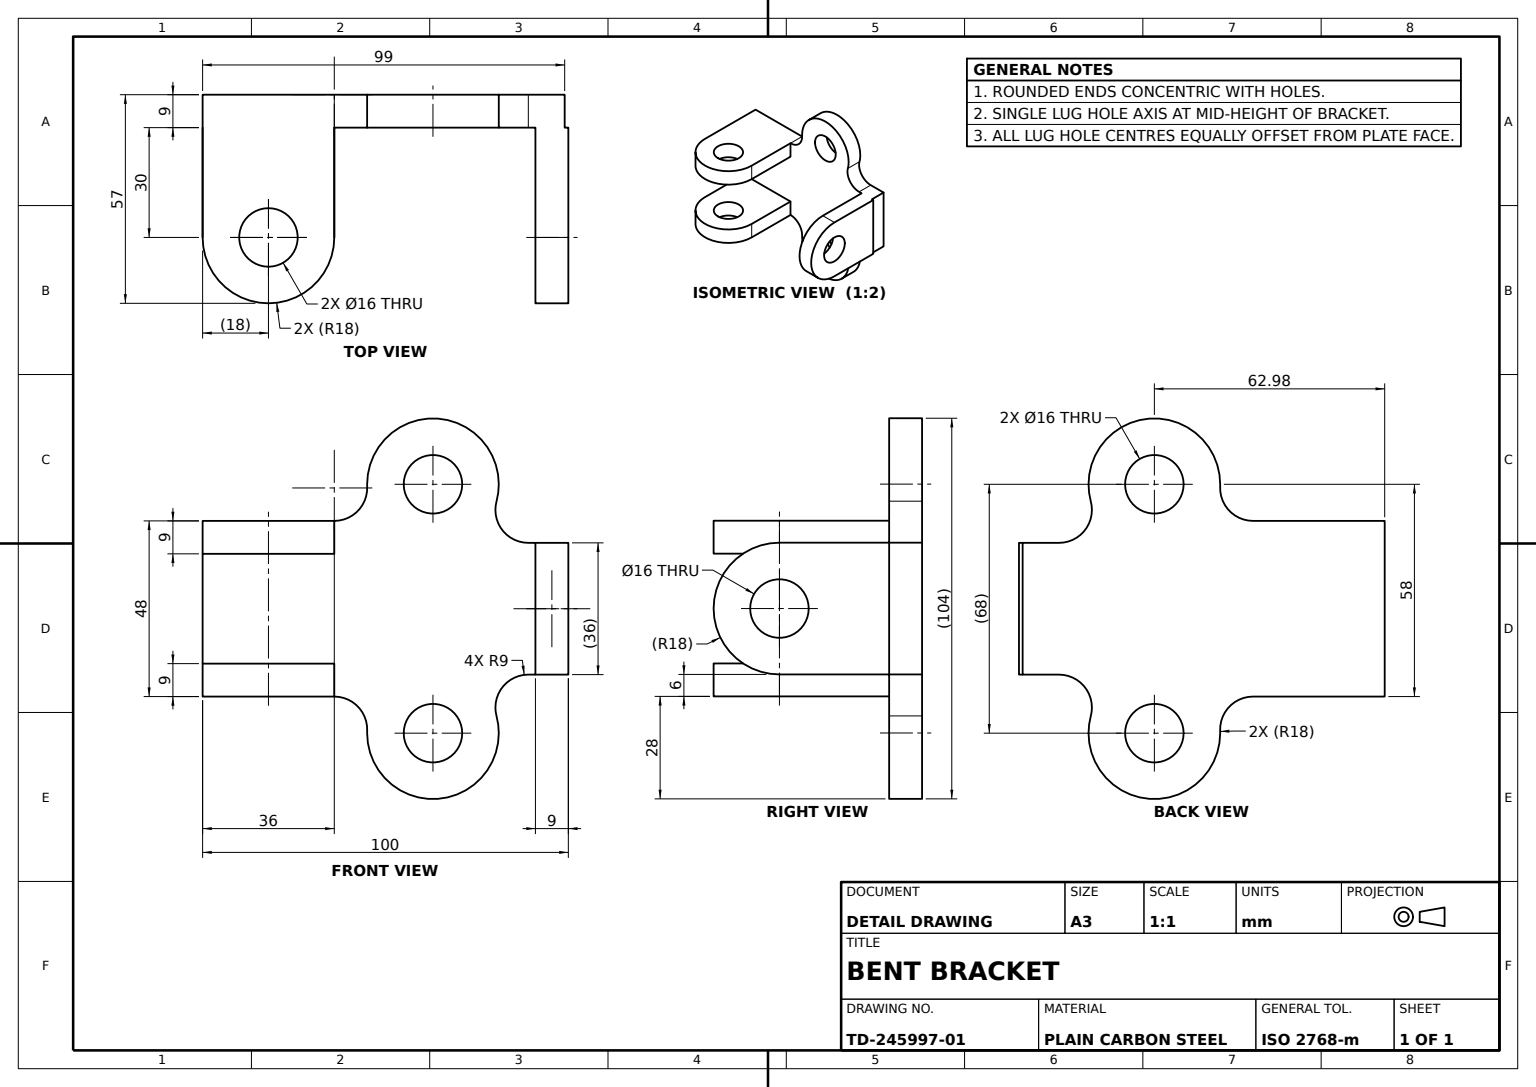
ISO-10303-21;
HEADER;
FILE_DESCRIPTION((''),'2;1');
FILE_NAME('','',(''),(''),'','','');
FILE_SCHEMA(('AUTOMOTIVE_DESIGN'));
ENDSEC;
DATA;
#1=APPLICATION_CONTEXT('');
#2=PRODUCT_CONTEXT('',#1,'mechanical');
#3=PRODUCT('','','',(#2));
#4=PRODUCT_DEFINITION_FORMATION('','',#3);
#5=PRODUCT_DEFINITION_CONTEXT('',#1,'design');
#6=PRODUCT_DEFINITION('','',#4,#5);
#7=PRODUCT_DEFINITION_SHAPE('','',#6);
#8=(LENGTH_UNIT()NAMED_UNIT(*)SI_UNIT(.MILLI.,.METRE.));
#9=(NAMED_UNIT(*)PLANE_ANGLE_UNIT()SI_UNIT($,.RADIAN.));
#10=(NAMED_UNIT(*)SI_UNIT($,.STERADIAN.)SOLID_ANGLE_UNIT());
#11=UNCERTAINTY_MEASURE_WITH_UNIT(LENGTH_MEASURE(1.E-05),#8,'distance_accuracy_value','');
#12=(GEOMETRIC_REPRESENTATION_CONTEXT(3)GLOBAL_UNCERTAINTY_ASSIGNED_CONTEXT((#11))GLOBAL_UNIT_ASSIGNED_CONTEXT((#8,#9,#10))REPRESENTATION_CONTEXT('',''));
#13=CARTESIAN_POINT('',(36.,9.,-30.));
#14=VERTEX_POINT('',#13);
#15=CARTESIAN_POINT('',(36.,0.,-30.));
#16=VERTEX_POINT('',#15);
#17=DIRECTION('',(0.,-1.,0.));
#18=VECTOR('',#17,1000.);
#19=LINE('',#13,#18);
#20=EDGE_CURVE('',#14,#16,#19,.T.);
#21=ORIENTED_EDGE('',*,*,#20,.F.);
#22=CARTESIAN_POINT('',(36.,9.,0.));
#23=VERTEX_POINT('',#22);
#24=DIRECTION('',(0.,0.,-1.));
#25=VECTOR('',#24,1000.);
#26=LINE('',#22,#25);
#27=EDGE_CURVE('',#23,#14,#26,.T.);
#28=ORIENTED_EDGE('',*,*,#27,.F.);
#29=CARTESIAN_POINT('',(36.,0.,0.));
#30=VERTEX_POINT('',#29);
#31=LINE('',#22,#18);
#32=EDGE_CURVE('',#23,#30,#31,.T.);
#33=ORIENTED_EDGE('',*,*,#32,.T.);
#34=LINE('',#29,#25);
#35=EDGE_CURVE('',#30,#16,#34,.T.);
#36=ORIENTED_EDGE('',*,*,#35,.T.);
#37=EDGE_LOOP('',(#21,#28,#33,#36));
#38=FACE_OUTER_BOUND('',#37,.T.);
#39=DIRECTION('',(-1.,0.,0.));
#40=DIRECTION('',(0.,0.,1.));
#41=AXIS2_PLACEMENT_3D('',#22,#39,#40);
#42=PLANE('',#41);
#43=ADVANCED_FACE('',(#38),#42,.F.);
#44=CARTESIAN_POINT('',(91.,24.,-22.));
#45=VERTEX_POINT('',#44);
#46=CARTESIAN_POINT('',(91.,24.,-38.));
#47=VERTEX_POINT('',#46);
#48=CARTESIAN_POINT('',(91.,24.,-30.));
#49=DIRECTION('',(1.,0.,0.));
#50=AXIS2_PLACEMENT_3D('',#48,#49,#24);
#51=CIRCLE('',#50,8.);
#52=EDGE_CURVE('',#45,#47,#51,.T.);
#53=ORIENTED_EDGE('',*,*,#52,.F.);
#54=CARTESIAN_POINT('',(100.,24.,-22.));
#55=VERTEX_POINT('',#54);
#56=VECTOR('',#49,1000.);
#57=LINE('',#44,#56);
#58=EDGE_CURVE('',#45,#55,#57,.T.);
#59=ORIENTED_EDGE('',*,*,#58,.T.);
#60=CARTESIAN_POINT('',(100.,24.,-38.));
#61=VERTEX_POINT('',#60);
#62=CARTESIAN_POINT('',(100.,24.,-30.));
#63=AXIS2_PLACEMENT_3D('',#62,#49,#24);
#64=CIRCLE('',#63,8.);
#65=EDGE_CURVE('',#55,#61,#64,.T.);
#66=ORIENTED_EDGE('',*,*,#65,.T.);
#67=LINE('',#46,#56);
#68=EDGE_CURVE('',#47,#61,#67,.T.);
#69=ORIENTED_EDGE('',*,*,#68,.F.);
#70=EDGE_LOOP('',(#53,#59,#66,#69));
#71=FACE_OUTER_BOUND('',#70,.T.);
#72=CYLINDRICAL_SURFACE('',#50,8.);
#73=ADVANCED_FACE('',(#71),#72,.F.);
#74=CARTESIAN_POINT('',(70.981475,-10.,9.));
#75=VERTEX_POINT('',#74);
#76=CARTESIAN_POINT('',(54.981475,-10.,9.));
#77=VERTEX_POINT('',#76);
#78=CARTESIAN_POINT('',(62.981475,-10.,9.));
#79=AXIS2_PLACEMENT_3D('',#78,#40,#49);
#80=CIRCLE('',#79,8.);
#81=EDGE_CURVE('',#75,#77,#80,.T.);
#82=ORIENTED_EDGE('',*,*,#81,.F.);
#83=EDGE_CURVE('',#77,#75,#80,.T.);
#84=ORIENTED_EDGE('',*,*,#83,.F.);
#85=EDGE_LOOP('',(#82,#84));
#86=FACE_BOUND('',#85,.T.);
#87=CARTESIAN_POINT('',(80.058285,51.,9.));
#88=VERTEX_POINT('',#87);
#89=CARTESIAN_POINT('',(80.366015,53.333333,9.));
#90=VERTEX_POINT('',#89);
#91=CARTESIAN_POINT('',(89.058285,51.,9.));
#92=AXIS2_PLACEMENT_3D('',#91,#24,#49);
#93=CIRCLE('',#92,9.);
#94=EDGE_CURVE('',#88,#90,#93,.T.);
#95=ORIENTED_EDGE('',*,*,#94,.T.);
#96=CARTESIAN_POINT('',(80.981475,58.,9.));
#97=VERTEX_POINT('',#96);
#98=CARTESIAN_POINT('',(62.981475,58.,9.));
#99=AXIS2_PLACEMENT_3D('',#98,#40,#49);
#100=CIRCLE('',#99,18.);
#101=EDGE_CURVE('',#90,#97,#100,.T.);
#102=ORIENTED_EDGE('',*,*,#101,.T.);
#103=CARTESIAN_POINT('',(44.981475,58.,9.));
#104=VERTEX_POINT('',#103);
#105=EDGE_CURVE('',#97,#104,#100,.T.);
#106=ORIENTED_EDGE('',*,*,#105,.T.);
#107=CARTESIAN_POINT('',(44.993825,57.333333,9.));
#108=VERTEX_POINT('',#107);
#109=EDGE_CURVE('',#104,#108,#100,.T.);
#110=ORIENTED_EDGE('',*,*,#109,.T.);
#111=CARTESIAN_POINT('',(36.,48.,9.));
#112=VERTEX_POINT('',#111);
#113=CARTESIAN_POINT('',(36.,57.,9.));
#114=AXIS2_PLACEMENT_3D('',#113,#24,#49);
#115=CIRCLE('',#114,9.);
#116=EDGE_CURVE('',#108,#112,#115,.T.);
#117=ORIENTED_EDGE('',*,*,#116,.T.);
#118=CARTESIAN_POINT('',(0.,48.,9.));
#119=VERTEX_POINT('',#118);
#120=VECTOR('',#39,1000.);
#121=LINE('',#118,#120);
#122=EDGE_CURVE('',#112,#119,#121,.T.);
#123=ORIENTED_EDGE('',*,*,#122,.T.);
#124=CARTESIAN_POINT('',(0.,0.,9.));
#125=VERTEX_POINT('',#124);
#126=LINE('',#124,#18);
#127=EDGE_CURVE('',#119,#125,#126,.T.);
#128=ORIENTED_EDGE('',*,*,#127,.T.);
#129=CARTESIAN_POINT('',(36.,0.,9.));
#130=VERTEX_POINT('',#129);
#131=LINE('',#124,#56);
#132=EDGE_CURVE('',#125,#130,#131,.T.);
#133=ORIENTED_EDGE('',*,*,#132,.T.);
#134=CARTESIAN_POINT('',(44.993825,-9.333333,9.));
#135=VERTEX_POINT('',#134);
#136=CARTESIAN_POINT('',(36.,-9.,9.));
#137=AXIS2_PLACEMENT_3D('',#136,#24,#49);
#138=CIRCLE('',#137,9.);
#139=EDGE_CURVE('',#130,#135,#138,.T.);
#140=ORIENTED_EDGE('',*,*,#139,.T.);
#141=CARTESIAN_POINT('',(44.981475,-10.,9.));
#142=VERTEX_POINT('',#141);
#143=CIRCLE('',#79,18.);
#144=EDGE_CURVE('',#135,#142,#143,.T.);
#145=ORIENTED_EDGE('',*,*,#144,.T.);
#146=CARTESIAN_POINT('',(80.981475,-10.,9.));
#147=VERTEX_POINT('',#146);
#148=EDGE_CURVE('',#142,#147,#143,.T.);
#149=ORIENTED_EDGE('',*,*,#148,.T.);
#150=CARTESIAN_POINT('',(80.366015,-5.333333,9.));
#151=VERTEX_POINT('',#150);
#152=EDGE_CURVE('',#147,#151,#143,.T.);
#153=ORIENTED_EDGE('',*,*,#152,.T.);
#154=CARTESIAN_POINT('',(80.058285,-3.,9.));
#155=VERTEX_POINT('',#154);
#156=CARTESIAN_POINT('',(89.058285,-3.,9.));
#157=AXIS2_PLACEMENT_3D('',#156,#24,#49);
#158=CIRCLE('',#157,9.);
#159=EDGE_CURVE('',#151,#155,#158,.T.);
#160=ORIENTED_EDGE('',*,*,#159,.T.);
#161=CARTESIAN_POINT('',(89.058285,6.,9.));
#162=VERTEX_POINT('',#161);
#163=EDGE_CURVE('',#155,#162,#158,.T.);
#164=ORIENTED_EDGE('',*,*,#163,.T.);
#165=CARTESIAN_POINT('',(99.,6.,9.));
#166=VERTEX_POINT('',#165);
#167=LINE('',#165,#56);
#168=EDGE_CURVE('',#162,#166,#167,.T.);
#169=ORIENTED_EDGE('',*,*,#168,.T.);
#170=CARTESIAN_POINT('',(99.,42.,9.));
#171=VERTEX_POINT('',#170);
#172=CARTESIAN_POINT('',(99.,24.,9.));
#173=DIRECTION('',(0.,1.,0.));
#174=VECTOR('',#173,1000.);
#175=LINE('',#172,#174);
#176=EDGE_CURVE('',#166,#171,#175,.T.);
#177=ORIENTED_EDGE('',*,*,#176,.T.);
#178=CARTESIAN_POINT('',(89.058285,42.,9.));
#179=VERTEX_POINT('',#178);
#180=LINE('',#170,#120);
#181=EDGE_CURVE('',#171,#179,#180,.T.);
#182=ORIENTED_EDGE('',*,*,#181,.T.);
#183=EDGE_CURVE('',#179,#88,#93,.T.);
#184=ORIENTED_EDGE('',*,*,#183,.T.);
#185=EDGE_LOOP('',(#95,#102,#106,#110,#117,#123,#128,#133,#140,#145,#149,#153,#160,#164,#169,#177,#182,#184));
#186=FACE_OUTER_BOUND('',#185,.T.);
#187=CARTESIAN_POINT('',(70.981475,58.,9.));
#188=VERTEX_POINT('',#187);
#189=CARTESIAN_POINT('',(54.981475,58.,9.));
#190=VERTEX_POINT('',#189);
#191=CIRCLE('',#99,8.);
#192=EDGE_CURVE('',#188,#190,#191,.T.);
#193=ORIENTED_EDGE('',*,*,#192,.F.);
#194=EDGE_CURVE('',#190,#188,#191,.T.);
#195=ORIENTED_EDGE('',*,*,#194,.F.);
#196=EDGE_LOOP('',(#193,#195));
#197=FACE_BOUND('',#196,.T.);
#198=AXIS2_PLACEMENT_3D('',#136,#40,#49);
#199=PLANE('',#198);
#200=ADVANCED_FACE('',(#86,#186,#197),#199,.T.);
#201=LINE('',#129,#25);
#202=EDGE_CURVE('',#130,#30,#201,.T.);
#203=ORIENTED_EDGE('',*,*,#202,.T.);
#204=CARTESIAN_POINT('',(44.993825,-9.333333,0.));
#205=VERTEX_POINT('',#204);
#206=CARTESIAN_POINT('',(36.,-9.,0.));
#207=AXIS2_PLACEMENT_3D('',#206,#24,#49);
#208=CIRCLE('',#207,9.);
#209=EDGE_CURVE('',#30,#205,#208,.T.);
#210=ORIENTED_EDGE('',*,*,#209,.T.);
#211=LINE('',#134,#25);
#212=EDGE_CURVE('',#135,#205,#211,.T.);
#213=ORIENTED_EDGE('',*,*,#212,.F.);
#214=ORIENTED_EDGE('',*,*,#139,.F.);
#215=EDGE_LOOP('',(#203,#210,#213,#214));
#216=FACE_OUTER_BOUND('',#215,.T.);
#217=AXIS2_PLACEMENT_3D('',#136,#24,#39);
#218=CYLINDRICAL_SURFACE('',#217,9.);
#219=ADVANCED_FACE('',(#216),#218,.F.);
#220=ORIENTED_EDGE('',*,*,#148,.F.);
#221=CARTESIAN_POINT('',(44.981475,-10.,0.));
#222=VERTEX_POINT('',#221);
#223=LINE('',#141,#25);
#224=EDGE_CURVE('',#142,#222,#223,.T.);
#225=ORIENTED_EDGE('',*,*,#224,.T.);
#226=CARTESIAN_POINT('',(80.981475,-10.,0.));
#227=VERTEX_POINT('',#226);
#228=CARTESIAN_POINT('',(62.981475,-10.,0.));
#229=AXIS2_PLACEMENT_3D('',#228,#40,#49);
#230=CIRCLE('',#229,18.);
#231=EDGE_CURVE('',#222,#227,#230,.T.);
#232=ORIENTED_EDGE('',*,*,#231,.T.);
#233=LINE('',#146,#25);
#234=EDGE_CURVE('',#147,#227,#233,.T.);
#235=ORIENTED_EDGE('',*,*,#234,.F.);
#236=EDGE_LOOP('',(#220,#225,#232,#235));
#237=FACE_OUTER_BOUND('',#236,.T.);
#238=AXIS2_PLACEMENT_3D('',#78,#24,#39);
#239=CYLINDRICAL_SURFACE('',#238,18.);
#240=ADVANCED_FACE('',(#237),#239,.T.);
#241=CARTESIAN_POINT('',(0.,9.,-30.));
#242=VERTEX_POINT('',#241);
#243=CARTESIAN_POINT('',(0.,0.,-30.));
#244=VERTEX_POINT('',#243);
#245=LINE('',#241,#18);
#246=EDGE_CURVE('',#242,#244,#245,.T.);
#247=ORIENTED_EDGE('',*,*,#246,.F.);
#248=CARTESIAN_POINT('',(18.,9.,-48.));
#249=VERTEX_POINT('',#248);
#250=CARTESIAN_POINT('',(18.,9.,-30.));
#251=AXIS2_PLACEMENT_3D('',#250,#173,#40);
#252=CIRCLE('',#251,18.);
#253=EDGE_CURVE('',#249,#242,#252,.T.);
#254=ORIENTED_EDGE('',*,*,#253,.F.);
#255=CARTESIAN_POINT('',(18.,0.,-48.));
#256=VERTEX_POINT('',#255);
#257=LINE('',#248,#18);
#258=EDGE_CURVE('',#249,#256,#257,.T.);
#259=ORIENTED_EDGE('',*,*,#258,.T.);
#260=CARTESIAN_POINT('',(18.,0.,-30.));
#261=AXIS2_PLACEMENT_3D('',#260,#173,#40);
#262=CIRCLE('',#261,18.);
#263=EDGE_CURVE('',#256,#244,#262,.T.);
#264=ORIENTED_EDGE('',*,*,#263,.T.);
#265=EDGE_LOOP('',(#247,#254,#259,#264));
#266=FACE_OUTER_BOUND('',#265,.T.);
#267=AXIS2_PLACEMENT_3D('',#250,#17,#24);
#268=CYLINDRICAL_SURFACE('',#267,18.);
#269=ADVANCED_FACE('',(#266),#268,.T.);
#270=CARTESIAN_POINT('',(80.366015,53.333333,0.));
#271=VERTEX_POINT('',#270);
#272=LINE('',#89,#25);
#273=EDGE_CURVE('',#90,#271,#272,.T.);
#274=ORIENTED_EDGE('',*,*,#273,.F.);
#275=ORIENTED_EDGE('',*,*,#94,.F.);
#276=CARTESIAN_POINT('',(80.058285,51.,0.));
#277=VERTEX_POINT('',#276);
#278=LINE('',#87,#25);
#279=EDGE_CURVE('',#88,#277,#278,.T.);
#280=ORIENTED_EDGE('',*,*,#279,.T.);
#281=CARTESIAN_POINT('',(89.058285,51.,0.));
#282=AXIS2_PLACEMENT_3D('',#281,#24,#49);
#283=CIRCLE('',#282,9.);
#284=EDGE_CURVE('',#277,#271,#283,.T.);
#285=ORIENTED_EDGE('',*,*,#284,.T.);
#286=EDGE_LOOP('',(#274,#275,#280,#285));
#287=FACE_OUTER_BOUND('',#286,.T.);
#288=AXIS2_PLACEMENT_3D('',#91,#24,#39);
#289=CYLINDRICAL_SURFACE('',#288,9.);
#290=ADVANCED_FACE('',(#287),#289,.F.);
#291=CARTESIAN_POINT('',(70.981475,58.,0.));
#292=VERTEX_POINT('',#291);
#293=LINE('',#187,#25);
#294=EDGE_CURVE('',#188,#292,#293,.T.);
#295=ORIENTED_EDGE('',*,*,#294,.T.);
#296=CARTESIAN_POINT('',(54.981475,58.,0.));
#297=VERTEX_POINT('',#296);
#298=CARTESIAN_POINT('',(62.981475,58.,0.));
#299=AXIS2_PLACEMENT_3D('',#298,#40,#49);
#300=CIRCLE('',#299,8.);
#301=EDGE_CURVE('',#297,#292,#300,.T.);
#302=ORIENTED_EDGE('',*,*,#301,.F.);
#303=LINE('',#189,#25);
#304=EDGE_CURVE('',#190,#297,#303,.T.);
#305=ORIENTED_EDGE('',*,*,#304,.F.);
#306=ORIENTED_EDGE('',*,*,#194,.T.);
#307=EDGE_LOOP('',(#295,#302,#305,#306));
#308=FACE_OUTER_BOUND('',#307,.T.);
#309=AXIS2_PLACEMENT_3D('',#98,#24,#39);
#310=CYLINDRICAL_SURFACE('',#309,8.);
#311=ADVANCED_FACE('',(#308),#310,.F.);
#312=ORIENTED_EDGE('',*,*,#181,.F.);
#313=CARTESIAN_POINT('',(99.,42.,0.));
#314=VERTEX_POINT('',#313);
#315=LINE('',#170,#25);
#316=EDGE_CURVE('',#171,#314,#315,.T.);
#317=ORIENTED_EDGE('',*,*,#316,.T.);
#318=CARTESIAN_POINT('',(100.,42.,0.));
#319=VERTEX_POINT('',#318);
#320=CARTESIAN_POINT('',(91.,42.,0.));
#321=LINE('',#320,#56);
#322=EDGE_CURVE('',#314,#319,#321,.T.);
#323=ORIENTED_EDGE('',*,*,#322,.T.);
#324=CARTESIAN_POINT('',(100.,42.,-30.));
#325=VERTEX_POINT('',#324);
#326=VECTOR('',#40,1000.);
#327=LINE('',#324,#326);
#328=EDGE_CURVE('',#325,#319,#327,.T.);
#329=ORIENTED_EDGE('',*,*,#328,.F.);
#330=CARTESIAN_POINT('',(91.,42.,-30.));
#331=VERTEX_POINT('',#330);
#332=LINE('',#330,#56);
#333=EDGE_CURVE('',#331,#325,#332,.T.);
#334=ORIENTED_EDGE('',*,*,#333,.F.);
#335=VERTEX_POINT('',#320);
#336=LINE('',#330,#326);
#337=EDGE_CURVE('',#331,#335,#336,.T.);
#338=ORIENTED_EDGE('',*,*,#337,.T.);
#339=CARTESIAN_POINT('',(89.058285,42.,0.));
#340=VERTEX_POINT('',#339);
#341=LINE('',#313,#120);
#342=EDGE_CURVE('',#335,#340,#341,.T.);
#343=ORIENTED_EDGE('',*,*,#342,.T.);
#344=LINE('',#178,#25);
#345=EDGE_CURVE('',#179,#340,#344,.T.);
#346=ORIENTED_EDGE('',*,*,#345,.F.);
#347=EDGE_LOOP('',(#312,#317,#323,#329,#334,#338,#343,#346));
#348=FACE_OUTER_BOUND('',#347,.T.);
#349=AXIS2_PLACEMENT_3D('',#170,#17,#24);
#350=PLANE('',#349);
#351=ADVANCED_FACE('',(#348),#350,.F.);
#352=CARTESIAN_POINT('',(36.,48.,0.));
#353=VERTEX_POINT('',#352);
#354=LINE('',#111,#25);
#355=EDGE_CURVE('',#112,#353,#354,.T.);
#356=ORIENTED_EDGE('',*,*,#355,.F.);
#357=ORIENTED_EDGE('',*,*,#116,.F.);
#358=CARTESIAN_POINT('',(44.993825,57.333333,0.));
#359=VERTEX_POINT('',#358);
#360=LINE('',#107,#25);
#361=EDGE_CURVE('',#108,#359,#360,.T.);
#362=ORIENTED_EDGE('',*,*,#361,.T.);
#363=CARTESIAN_POINT('',(36.,57.,0.));
#364=AXIS2_PLACEMENT_3D('',#363,#24,#49);
#365=CIRCLE('',#364,9.);
#366=EDGE_CURVE('',#359,#353,#365,.T.);
#367=ORIENTED_EDGE('',*,*,#366,.T.);
#368=EDGE_LOOP('',(#356,#357,#362,#367));
#369=FACE_OUTER_BOUND('',#368,.T.);
#370=AXIS2_PLACEMENT_3D('',#113,#24,#39);
#371=CYLINDRICAL_SURFACE('',#370,9.);
#372=ADVANCED_FACE('',(#369),#371,.F.);
#373=CARTESIAN_POINT('',(100.,24.,-48.));
#374=VERTEX_POINT('',#373);
#375=CIRCLE('',#63,18.);
#376=EDGE_CURVE('',#374,#325,#375,.T.);
#377=ORIENTED_EDGE('',*,*,#376,.F.);
#378=CARTESIAN_POINT('',(91.,24.,-48.));
#379=VERTEX_POINT('',#378);
#380=LINE('',#378,#56);
#381=EDGE_CURVE('',#379,#374,#380,.T.);
#382=ORIENTED_EDGE('',*,*,#381,.F.);
#383=CIRCLE('',#50,18.);
#384=EDGE_CURVE('',#379,#331,#383,.T.);
#385=ORIENTED_EDGE('',*,*,#384,.T.);
#386=ORIENTED_EDGE('',*,*,#333,.T.);
#387=EDGE_LOOP('',(#377,#382,#385,#386));
#388=FACE_OUTER_BOUND('',#387,.T.);
#389=CYLINDRICAL_SURFACE('',#50,18.);
#390=ADVANCED_FACE('',(#388),#389,.T.);
#391=ORIENTED_EDGE('',*,*,#35,.F.);
#392=ORIENTED_EDGE('',*,*,#202,.F.);
#393=ORIENTED_EDGE('',*,*,#132,.F.);
#394=LINE('',#124,#25);
#395=EDGE_CURVE('',#125,#244,#394,.T.);
#396=ORIENTED_EDGE('',*,*,#395,.T.);
#397=ORIENTED_EDGE('',*,*,#263,.F.);
#398=EDGE_CURVE('',#16,#256,#262,.T.);
#399=ORIENTED_EDGE('',*,*,#398,.F.);
#400=EDGE_LOOP('',(#391,#392,#393,#396,#397,#399));
#401=FACE_OUTER_BOUND('',#400,.T.);
#402=CARTESIAN_POINT('',(18.,0.,-38.));
#403=VERTEX_POINT('',#402);
#404=CARTESIAN_POINT('',(18.,0.,-22.));
#405=VERTEX_POINT('',#404);
#406=CIRCLE('',#261,8.);
#407=EDGE_CURVE('',#403,#405,#406,.T.);
#408=ORIENTED_EDGE('',*,*,#407,.T.);
#409=EDGE_CURVE('',#405,#403,#406,.T.);
#410=ORIENTED_EDGE('',*,*,#409,.T.);
#411=EDGE_LOOP('',(#408,#410));
#412=FACE_BOUND('',#411,.T.);
#413=AXIS2_PLACEMENT_3D('',#124,#173,#40);
#414=PLANE('',#413);
#415=ADVANCED_FACE('',(#401,#412),#414,.F.);
#416=ORIENTED_EDGE('',*,*,#301,.T.);
#417=EDGE_CURVE('',#292,#297,#300,.T.);
#418=ORIENTED_EDGE('',*,*,#417,.T.);
#419=EDGE_LOOP('',(#416,#418));
#420=FACE_BOUND('',#419,.T.);
#421=CARTESIAN_POINT('',(70.981475,-10.,0.));
#422=VERTEX_POINT('',#421);
#423=CARTESIAN_POINT('',(54.981475,-10.,0.));
#424=VERTEX_POINT('',#423);
#425=CIRCLE('',#229,8.);
#426=EDGE_CURVE('',#422,#424,#425,.T.);
#427=ORIENTED_EDGE('',*,*,#426,.T.);
#428=EDGE_CURVE('',#424,#422,#425,.T.);
#429=ORIENTED_EDGE('',*,*,#428,.T.);
#430=EDGE_LOOP('',(#427,#429));
#431=FACE_BOUND('',#430,.T.);
#432=CARTESIAN_POINT('',(0.,39.,0.));
#433=VERTEX_POINT('',#432);
#434=CARTESIAN_POINT('',(0.,9.,0.));
#435=VERTEX_POINT('',#434);
#436=CARTESIAN_POINT('',(0.,0.,0.));
#437=LINE('',#436,#18);
#438=EDGE_CURVE('',#433,#435,#437,.T.);
#439=ORIENTED_EDGE('',*,*,#438,.F.);
#440=CARTESIAN_POINT('',(36.,39.,0.));
#441=VERTEX_POINT('',#440);
#442=LINE('',#432,#56);
#443=EDGE_CURVE('',#433,#441,#442,.T.);
#444=ORIENTED_EDGE('',*,*,#443,.T.);
#445=LINE('',#440,#174);
#446=EDGE_CURVE('',#441,#353,#445,.T.);
#447=ORIENTED_EDGE('',*,*,#446,.T.);
#448=ORIENTED_EDGE('',*,*,#366,.F.);
#449=CARTESIAN_POINT('',(44.981475,58.,0.));
#450=VERTEX_POINT('',#449);
#451=CIRCLE('',#299,18.);
#452=EDGE_CURVE('',#450,#359,#451,.T.);
#453=ORIENTED_EDGE('',*,*,#452,.F.);
#454=CARTESIAN_POINT('',(80.981475,58.,0.));
#455=VERTEX_POINT('',#454);
#456=EDGE_CURVE('',#455,#450,#451,.T.);
#457=ORIENTED_EDGE('',*,*,#456,.F.);
#458=EDGE_CURVE('',#271,#455,#451,.T.);
#459=ORIENTED_EDGE('',*,*,#458,.F.);
#460=ORIENTED_EDGE('',*,*,#284,.F.);
#461=EDGE_CURVE('',#340,#277,#283,.T.);
#462=ORIENTED_EDGE('',*,*,#461,.F.);
#463=ORIENTED_EDGE('',*,*,#342,.F.);
#464=CARTESIAN_POINT('',(91.,6.,0.));
#465=VERTEX_POINT('',#464);
#466=LINE('',#320,#18);
#467=EDGE_CURVE('',#335,#465,#466,.T.);
#468=ORIENTED_EDGE('',*,*,#467,.T.);
#469=CARTESIAN_POINT('',(89.058285,6.,0.));
#470=VERTEX_POINT('',#469);
#471=CARTESIAN_POINT('',(99.,6.,0.));
#472=LINE('',#471,#56);
#473=EDGE_CURVE('',#470,#465,#472,.T.);
#474=ORIENTED_EDGE('',*,*,#473,.F.);
#475=CARTESIAN_POINT('',(80.058285,-3.,0.));
#476=VERTEX_POINT('',#475);
#477=CARTESIAN_POINT('',(89.058285,-3.,0.));
#478=AXIS2_PLACEMENT_3D('',#477,#24,#49);
#479=CIRCLE('',#478,9.);
#480=EDGE_CURVE('',#476,#470,#479,.T.);
#481=ORIENTED_EDGE('',*,*,#480,.F.);
#482=CARTESIAN_POINT('',(80.366015,-5.333333,0.));
#483=VERTEX_POINT('',#482);
#484=EDGE_CURVE('',#483,#476,#479,.T.);
#485=ORIENTED_EDGE('',*,*,#484,.F.);
#486=EDGE_CURVE('',#227,#483,#230,.T.);
#487=ORIENTED_EDGE('',*,*,#486,.F.);
#488=ORIENTED_EDGE('',*,*,#231,.F.);
#489=EDGE_CURVE('',#205,#222,#230,.T.);
#490=ORIENTED_EDGE('',*,*,#489,.F.);
#491=ORIENTED_EDGE('',*,*,#209,.F.);
#492=ORIENTED_EDGE('',*,*,#32,.F.);
#493=LINE('',#434,#56);
#494=EDGE_CURVE('',#435,#23,#493,.T.);
#495=ORIENTED_EDGE('',*,*,#494,.F.);
#496=EDGE_LOOP('',(#439,#444,#447,#448,#453,#457,#459,#460,#462,#463,#468,#474,#481,#485,#487,#488,#490,#491,#492,#495));
#497=FACE_OUTER_BOUND('',#496,.T.);
#498=AXIS2_PLACEMENT_3D('',#206,#40,#49);
#499=PLANE('',#498);
#500=ADVANCED_FACE('',(#420,#431,#497),#499,.F.);
#501=ORIENTED_EDGE('',*,*,#361,.F.);
#502=ORIENTED_EDGE('',*,*,#109,.F.);
#503=LINE('',#103,#25);
#504=EDGE_CURVE('',#104,#450,#503,.T.);
#505=ORIENTED_EDGE('',*,*,#504,.T.);
#506=ORIENTED_EDGE('',*,*,#452,.T.);
#507=EDGE_LOOP('',(#501,#502,#505,#506));
#508=FACE_OUTER_BOUND('',#507,.T.);
#509=CYLINDRICAL_SURFACE('',#309,18.);
#510=ADVANCED_FACE('',(#508),#509,.T.);
#511=CARTESIAN_POINT('',(18.,9.,-22.));
#512=VERTEX_POINT('',#511);
#513=CARTESIAN_POINT('',(18.,9.,-38.));
#514=VERTEX_POINT('',#513);
#515=CIRCLE('',#251,8.);
#516=EDGE_CURVE('',#512,#514,#515,.T.);
#517=ORIENTED_EDGE('',*,*,#516,.F.);
#518=EDGE_CURVE('',#514,#512,#515,.T.);
#519=ORIENTED_EDGE('',*,*,#518,.F.);
#520=EDGE_LOOP('',(#517,#519));
#521=FACE_BOUND('',#520,.T.);
#522=ORIENTED_EDGE('',*,*,#27,.T.);
#523=EDGE_CURVE('',#14,#249,#252,.T.);
#524=ORIENTED_EDGE('',*,*,#523,.T.);
#525=ORIENTED_EDGE('',*,*,#253,.T.);
#526=LINE('',#241,#326);
#527=EDGE_CURVE('',#242,#435,#526,.T.);
#528=ORIENTED_EDGE('',*,*,#527,.T.);
#529=ORIENTED_EDGE('',*,*,#494,.T.);
#530=EDGE_LOOP('',(#522,#524,#525,#528,#529));
#531=FACE_OUTER_BOUND('',#530,.T.);
#532=PLANE('',#251);
#533=ADVANCED_FACE('',(#521,#531),#532,.T.);
#534=LINE('',#96,#25);
#535=EDGE_CURVE('',#97,#455,#534,.T.);
#536=ORIENTED_EDGE('',*,*,#535,.F.);
#537=ORIENTED_EDGE('',*,*,#101,.F.);
#538=ORIENTED_EDGE('',*,*,#273,.T.);
#539=ORIENTED_EDGE('',*,*,#458,.T.);
#540=EDGE_LOOP('',(#536,#537,#538,#539));
#541=FACE_OUTER_BOUND('',#540,.T.);
#542=ADVANCED_FACE('',(#541),#509,.T.);
#543=ORIENTED_EDGE('',*,*,#384,.F.);
#544=CARTESIAN_POINT('',(91.,6.,-30.));
#545=VERTEX_POINT('',#544);
#546=EDGE_CURVE('',#545,#379,#383,.T.);
#547=ORIENTED_EDGE('',*,*,#546,.F.);
#548=LINE('',#464,#25);
#549=EDGE_CURVE('',#465,#545,#548,.T.);
#550=ORIENTED_EDGE('',*,*,#549,.F.);
#551=ORIENTED_EDGE('',*,*,#467,.F.);
#552=ORIENTED_EDGE('',*,*,#337,.F.);
#553=EDGE_LOOP('',(#543,#547,#550,#551,#552));
#554=FACE_OUTER_BOUND('',#553,.T.);
#555=EDGE_CURVE('',#47,#45,#51,.T.);
#556=ORIENTED_EDGE('',*,*,#555,.T.);
#557=ORIENTED_EDGE('',*,*,#52,.T.);
#558=EDGE_LOOP('',(#556,#557));
#559=FACE_BOUND('',#558,.T.);
#560=PLANE('',#50);
#561=ADVANCED_FACE('',(#554,#559),#560,.F.);
#562=CARTESIAN_POINT('',(0.,48.,-30.));
#563=VERTEX_POINT('',#562);
#564=LINE('',#118,#25);
#565=EDGE_CURVE('',#119,#563,#564,.T.);
#566=ORIENTED_EDGE('',*,*,#565,.T.);
#567=CARTESIAN_POINT('',(0.,39.,-30.));
#568=VERTEX_POINT('',#567);
#569=LINE('',#567,#174);
#570=EDGE_CURVE('',#568,#563,#569,.T.);
#571=ORIENTED_EDGE('',*,*,#570,.F.);
#572=LINE('',#567,#326);
#573=EDGE_CURVE('',#568,#433,#572,.T.);
#574=ORIENTED_EDGE('',*,*,#573,.T.);
#575=ORIENTED_EDGE('',*,*,#438,.T.);
#576=ORIENTED_EDGE('',*,*,#527,.F.);
#577=ORIENTED_EDGE('',*,*,#246,.T.);
#578=ORIENTED_EDGE('',*,*,#395,.F.);
#579=ORIENTED_EDGE('',*,*,#127,.F.);
#580=EDGE_LOOP('',(#566,#571,#574,#575,#576,#577,#578,#579));
#581=FACE_OUTER_BOUND('',#580,.T.);
#582=AXIS2_PLACEMENT_3D('',#124,#49,#24);
#583=PLANE('',#582);
#584=ADVANCED_FACE('',(#581),#583,.F.);
#585=ORIENTED_EDGE('',*,*,#504,.F.);
#586=ORIENTED_EDGE('',*,*,#105,.F.);
#587=ORIENTED_EDGE('',*,*,#535,.T.);
#588=ORIENTED_EDGE('',*,*,#456,.T.);
#589=EDGE_LOOP('',(#585,#586,#587,#588));
#590=FACE_OUTER_BOUND('',#589,.T.);
#591=ADVANCED_FACE('',(#590),#509,.T.);
#592=ORIENTED_EDGE('',*,*,#176,.F.);
#593=VERTEX_POINT('',#471);
#594=LINE('',#165,#25);
#595=EDGE_CURVE('',#166,#593,#594,.T.);
#596=ORIENTED_EDGE('',*,*,#595,.T.);
#597=CARTESIAN_POINT('',(99.,24.,0.));
#598=LINE('',#597,#174);
#599=EDGE_CURVE('',#593,#314,#598,.T.);
#600=ORIENTED_EDGE('',*,*,#599,.T.);
#601=ORIENTED_EDGE('',*,*,#316,.F.);
#602=EDGE_LOOP('',(#592,#596,#600,#601));
#603=FACE_OUTER_BOUND('',#602,.T.);
#604=AXIS2_PLACEMENT_3D('',#172,#39,#40);
#605=PLANE('',#604);
#606=ADVANCED_FACE('',(#603),#605,.F.);
#607=ORIENTED_EDGE('',*,*,#192,.T.);
#608=ORIENTED_EDGE('',*,*,#304,.T.);
#609=ORIENTED_EDGE('',*,*,#417,.F.);
#610=ORIENTED_EDGE('',*,*,#294,.F.);
#611=EDGE_LOOP('',(#607,#608,#609,#610));
#612=FACE_OUTER_BOUND('',#611,.T.);
#613=ADVANCED_FACE('',(#612),#310,.F.);
#614=ORIENTED_EDGE('',*,*,#446,.F.);
#615=CARTESIAN_POINT('',(36.,39.,-30.));
#616=VERTEX_POINT('',#615);
#617=LINE('',#440,#25);
#618=EDGE_CURVE('',#441,#616,#617,.T.);
#619=ORIENTED_EDGE('',*,*,#618,.T.);
#620=CARTESIAN_POINT('',(36.,48.,-30.));
#621=VERTEX_POINT('',#620);
#622=LINE('',#615,#174);
#623=EDGE_CURVE('',#616,#621,#622,.T.);
#624=ORIENTED_EDGE('',*,*,#623,.T.);
#625=LINE('',#352,#25);
#626=EDGE_CURVE('',#353,#621,#625,.T.);
#627=ORIENTED_EDGE('',*,*,#626,.F.);
#628=EDGE_LOOP('',(#614,#619,#624,#627));
#629=FACE_OUTER_BOUND('',#628,.T.);
#630=AXIS2_PLACEMENT_3D('',#440,#49,#24);
#631=PLANE('',#630);
#632=ADVANCED_FACE('',(#629),#631,.T.);
#633=ORIENTED_EDGE('',*,*,#183,.F.);
#634=ORIENTED_EDGE('',*,*,#345,.T.);
#635=ORIENTED_EDGE('',*,*,#461,.T.);
#636=ORIENTED_EDGE('',*,*,#279,.F.);
#637=EDGE_LOOP('',(#633,#634,#635,#636));
#638=FACE_OUTER_BOUND('',#637,.T.);
#639=ADVANCED_FACE('',(#638),#289,.F.);
#640=ORIENTED_EDGE('',*,*,#565,.F.);
#641=ORIENTED_EDGE('',*,*,#122,.F.);
#642=ORIENTED_EDGE('',*,*,#355,.T.);
#643=ORIENTED_EDGE('',*,*,#626,.T.);
#644=CARTESIAN_POINT('',(18.,48.,-30.));
#645=AXIS2_PLACEMENT_3D('',#644,#173,#40);
#646=CIRCLE('',#645,18.);
#647=EDGE_CURVE('',#621,#563,#646,.T.);
#648=ORIENTED_EDGE('',*,*,#647,.T.);
#649=EDGE_LOOP('',(#640,#641,#642,#643,#648));
#650=FACE_OUTER_BOUND('',#649,.T.);
#651=CARTESIAN_POINT('',(18.,48.,-38.));
#652=VERTEX_POINT('',#651);
#653=CARTESIAN_POINT('',(18.,48.,-22.));
#654=VERTEX_POINT('',#653);
#655=CIRCLE('',#645,8.);
#656=EDGE_CURVE('',#652,#654,#655,.T.);
#657=ORIENTED_EDGE('',*,*,#656,.F.);
#658=EDGE_CURVE('',#654,#652,#655,.T.);
#659=ORIENTED_EDGE('',*,*,#658,.F.);
#660=EDGE_LOOP('',(#657,#659));
#661=FACE_BOUND('',#660,.T.);
#662=AXIS2_PLACEMENT_3D('',#118,#17,#49);
#663=PLANE('',#662);
#664=ADVANCED_FACE('',(#650,#661),#663,.F.);
#665=ORIENTED_EDGE('',*,*,#546,.T.);
#666=ORIENTED_EDGE('',*,*,#381,.T.);
#667=CARTESIAN_POINT('',(100.,6.,-30.));
#668=VERTEX_POINT('',#667);
#669=EDGE_CURVE('',#668,#374,#375,.T.);
#670=ORIENTED_EDGE('',*,*,#669,.F.);
#671=LINE('',#544,#56);
#672=EDGE_CURVE('',#545,#668,#671,.T.);
#673=ORIENTED_EDGE('',*,*,#672,.F.);
#674=EDGE_LOOP('',(#665,#666,#670,#673));
#675=FACE_OUTER_BOUND('',#674,.T.);
#676=ADVANCED_FACE('',(#675),#389,.T.);
#677=ORIENTED_EDGE('',*,*,#595,.F.);
#678=ORIENTED_EDGE('',*,*,#168,.F.);
#679=LINE('',#161,#25);
#680=EDGE_CURVE('',#162,#470,#679,.T.);
#681=ORIENTED_EDGE('',*,*,#680,.T.);
#682=ORIENTED_EDGE('',*,*,#473,.T.);
#683=ORIENTED_EDGE('',*,*,#549,.T.);
#684=ORIENTED_EDGE('',*,*,#672,.T.);
#685=CARTESIAN_POINT('',(100.,6.,0.));
#686=VERTEX_POINT('',#685);
#687=LINE('',#685,#25);
#688=EDGE_CURVE('',#686,#668,#687,.T.);
#689=ORIENTED_EDGE('',*,*,#688,.F.);
#690=LINE('',#464,#56);
#691=EDGE_CURVE('',#593,#686,#690,.T.);
#692=ORIENTED_EDGE('',*,*,#691,.F.);
#693=EDGE_LOOP('',(#677,#678,#681,#682,#683,#684,#689,#692));
#694=FACE_OUTER_BOUND('',#693,.T.);
#695=AXIS2_PLACEMENT_3D('',#165,#173,#39);
#696=PLANE('',#695);
#697=ADVANCED_FACE('',(#694),#696,.F.);
#698=CARTESIAN_POINT('',(18.,39.,-30.));
#699=AXIS2_PLACEMENT_3D('',#698,#173,#40);
#700=CIRCLE('',#699,18.);
#701=EDGE_CURVE('',#616,#568,#700,.T.);
#702=ORIENTED_EDGE('',*,*,#701,.F.);
#703=ORIENTED_EDGE('',*,*,#618,.F.);
#704=ORIENTED_EDGE('',*,*,#443,.F.);
#705=ORIENTED_EDGE('',*,*,#573,.F.);
#706=EDGE_LOOP('',(#702,#703,#704,#705));
#707=FACE_OUTER_BOUND('',#706,.T.);
#708=CARTESIAN_POINT('',(18.,39.,-38.));
#709=VERTEX_POINT('',#708);
#710=CARTESIAN_POINT('',(18.,39.,-22.));
#711=VERTEX_POINT('',#710);
#712=CIRCLE('',#699,8.);
#713=EDGE_CURVE('',#709,#711,#712,.T.);
#714=ORIENTED_EDGE('',*,*,#713,.T.);
#715=EDGE_CURVE('',#711,#709,#712,.T.);
#716=ORIENTED_EDGE('',*,*,#715,.T.);
#717=EDGE_LOOP('',(#714,#716));
#718=FACE_BOUND('',#717,.T.);
#719=PLANE('',#699);
#720=ADVANCED_FACE('',(#707,#718),#719,.F.);
#721=ORIENTED_EDGE('',*,*,#489,.T.);
#722=ORIENTED_EDGE('',*,*,#224,.F.);
#723=ORIENTED_EDGE('',*,*,#144,.F.);
#724=ORIENTED_EDGE('',*,*,#212,.T.);
#725=EDGE_LOOP('',(#721,#722,#723,#724));
#726=FACE_OUTER_BOUND('',#725,.T.);
#727=ADVANCED_FACE('',(#726),#239,.T.);
#728=LINE('',#150,#25);
#729=EDGE_CURVE('',#151,#483,#728,.T.);
#730=ORIENTED_EDGE('',*,*,#729,.F.);
#731=ORIENTED_EDGE('',*,*,#152,.F.);
#732=ORIENTED_EDGE('',*,*,#234,.T.);
#733=ORIENTED_EDGE('',*,*,#486,.T.);
#734=EDGE_LOOP('',(#730,#731,#732,#733));
#735=FACE_OUTER_BOUND('',#734,.T.);
#736=ADVANCED_FACE('',(#735),#239,.T.);
#737=ORIENTED_EDGE('',*,*,#555,.F.);
#738=ORIENTED_EDGE('',*,*,#68,.T.);
#739=EDGE_CURVE('',#61,#55,#64,.T.);
#740=ORIENTED_EDGE('',*,*,#739,.T.);
#741=ORIENTED_EDGE('',*,*,#58,.F.);
#742=EDGE_LOOP('',(#737,#738,#740,#741));
#743=FACE_OUTER_BOUND('',#742,.T.);
#744=ADVANCED_FACE('',(#743),#72,.F.);
#745=ORIENTED_EDGE('',*,*,#83,.T.);
#746=LINE('',#74,#25);
#747=EDGE_CURVE('',#75,#422,#746,.T.);
#748=ORIENTED_EDGE('',*,*,#747,.T.);
#749=ORIENTED_EDGE('',*,*,#428,.F.);
#750=LINE('',#76,#25);
#751=EDGE_CURVE('',#77,#424,#750,.T.);
#752=ORIENTED_EDGE('',*,*,#751,.F.);
#753=EDGE_LOOP('',(#745,#748,#749,#752));
#754=FACE_OUTER_BOUND('',#753,.T.);
#755=CYLINDRICAL_SURFACE('',#238,8.);
#756=ADVANCED_FACE('',(#754),#755,.F.);
#757=ORIENTED_EDGE('',*,*,#163,.F.);
#758=LINE('',#154,#25);
#759=EDGE_CURVE('',#155,#476,#758,.T.);
#760=ORIENTED_EDGE('',*,*,#759,.T.);
#761=ORIENTED_EDGE('',*,*,#480,.T.);
#762=ORIENTED_EDGE('',*,*,#680,.F.);
#763=EDGE_LOOP('',(#757,#760,#761,#762));
#764=FACE_OUTER_BOUND('',#763,.T.);
#765=AXIS2_PLACEMENT_3D('',#156,#24,#39);
#766=CYLINDRICAL_SURFACE('',#765,9.);
#767=ADVANCED_FACE('',(#764),#766,.F.);
#768=ORIENTED_EDGE('',*,*,#701,.T.);
#769=ORIENTED_EDGE('',*,*,#570,.T.);
#770=ORIENTED_EDGE('',*,*,#647,.F.);
#771=ORIENTED_EDGE('',*,*,#623,.F.);
#772=EDGE_LOOP('',(#768,#769,#770,#771));
#773=FACE_OUTER_BOUND('',#772,.T.);
#774=CYLINDRICAL_SURFACE('',#699,18.);
#775=ADVANCED_FACE('',(#773),#774,.T.);
#776=ORIENTED_EDGE('',*,*,#407,.F.);
#777=LINE('',#513,#18);
#778=EDGE_CURVE('',#514,#403,#777,.T.);
#779=ORIENTED_EDGE('',*,*,#778,.F.);
#780=ORIENTED_EDGE('',*,*,#518,.T.);
#781=LINE('',#511,#18);
#782=EDGE_CURVE('',#512,#405,#781,.T.);
#783=ORIENTED_EDGE('',*,*,#782,.T.);
#784=EDGE_LOOP('',(#776,#779,#780,#783));
#785=FACE_OUTER_BOUND('',#784,.T.);
#786=CYLINDRICAL_SURFACE('',#267,8.);
#787=ADVANCED_FACE('',(#785),#786,.F.);
#788=ORIENTED_EDGE('',*,*,#409,.F.);
#789=ORIENTED_EDGE('',*,*,#782,.F.);
#790=ORIENTED_EDGE('',*,*,#516,.T.);
#791=ORIENTED_EDGE('',*,*,#778,.T.);
#792=EDGE_LOOP('',(#788,#789,#790,#791));
#793=FACE_OUTER_BOUND('',#792,.T.);
#794=ADVANCED_FACE('',(#793),#786,.F.);
#795=LINE('',#708,#174);
#796=EDGE_CURVE('',#709,#652,#795,.T.);
#797=ORIENTED_EDGE('',*,*,#796,.T.);
#798=ORIENTED_EDGE('',*,*,#656,.T.);
#799=LINE('',#710,#174);
#800=EDGE_CURVE('',#711,#654,#799,.T.);
#801=ORIENTED_EDGE('',*,*,#800,.F.);
#802=ORIENTED_EDGE('',*,*,#713,.F.);
#803=EDGE_LOOP('',(#797,#798,#801,#802));
#804=FACE_OUTER_BOUND('',#803,.T.);
#805=CYLINDRICAL_SURFACE('',#699,8.);
#806=ADVANCED_FACE('',(#804),#805,.F.);
#807=ORIENTED_EDGE('',*,*,#258,.F.);
#808=ORIENTED_EDGE('',*,*,#523,.F.);
#809=ORIENTED_EDGE('',*,*,#20,.T.);
#810=ORIENTED_EDGE('',*,*,#398,.T.);
#811=EDGE_LOOP('',(#807,#808,#809,#810));
#812=FACE_OUTER_BOUND('',#811,.T.);
#813=ADVANCED_FACE('',(#812),#268,.T.);
#814=LINE('',#318,#18);
#815=EDGE_CURVE('',#319,#686,#814,.T.);
#816=ORIENTED_EDGE('',*,*,#815,.T.);
#817=ORIENTED_EDGE('',*,*,#688,.T.);
#818=ORIENTED_EDGE('',*,*,#669,.T.);
#819=ORIENTED_EDGE('',*,*,#376,.T.);
#820=ORIENTED_EDGE('',*,*,#328,.T.);
#821=EDGE_LOOP('',(#816,#817,#818,#819,#820));
#822=FACE_OUTER_BOUND('',#821,.T.);
#823=ORIENTED_EDGE('',*,*,#65,.F.);
#824=ORIENTED_EDGE('',*,*,#739,.F.);
#825=EDGE_LOOP('',(#823,#824));
#826=FACE_BOUND('',#825,.T.);
#827=PLANE('',#63);
#828=ADVANCED_FACE('',(#822,#826),#827,.T.);
#829=ORIENTED_EDGE('',*,*,#426,.F.);
#830=ORIENTED_EDGE('',*,*,#747,.F.);
#831=ORIENTED_EDGE('',*,*,#81,.T.);
#832=ORIENTED_EDGE('',*,*,#751,.T.);
#833=EDGE_LOOP('',(#829,#830,#831,#832));
#834=FACE_OUTER_BOUND('',#833,.T.);
#835=ADVANCED_FACE('',(#834),#755,.F.);
#836=ORIENTED_EDGE('',*,*,#815,.F.);
#837=ORIENTED_EDGE('',*,*,#322,.F.);
#838=ORIENTED_EDGE('',*,*,#599,.F.);
#839=ORIENTED_EDGE('',*,*,#691,.T.);
#840=EDGE_LOOP('',(#836,#837,#838,#839));
#841=FACE_OUTER_BOUND('',#840,.T.);
#842=AXIS2_PLACEMENT_3D('',#320,#40,#49);
#843=PLANE('',#842);
#844=ADVANCED_FACE('',(#841),#843,.T.);
#845=ORIENTED_EDGE('',*,*,#159,.F.);
#846=ORIENTED_EDGE('',*,*,#729,.T.);
#847=ORIENTED_EDGE('',*,*,#484,.T.);
#848=ORIENTED_EDGE('',*,*,#759,.F.);
#849=EDGE_LOOP('',(#845,#846,#847,#848));
#850=FACE_OUTER_BOUND('',#849,.T.);
#851=ADVANCED_FACE('',(#850),#766,.F.);
#852=ORIENTED_EDGE('',*,*,#715,.F.);
#853=ORIENTED_EDGE('',*,*,#800,.T.);
#854=ORIENTED_EDGE('',*,*,#658,.T.);
#855=ORIENTED_EDGE('',*,*,#796,.F.);
#856=EDGE_LOOP('',(#852,#853,#854,#855));
#857=FACE_OUTER_BOUND('',#856,.T.);
#858=ADVANCED_FACE('',(#857),#805,.F.);
#859=CLOSED_SHELL('',(#43,#73,#200,#219,#240,#269,#290,#311,#351,#372,#390,#415,#500,#510,#533,#542,#561,#584,#591,#606,#613,#632,#639,#664,#676,#697,#720,#727,#736,#744,#756,#767,#775,#787,#794,#806,#813,#828,#835,#844,#851,#858));
#860=MANIFOLD_SOLID_BREP('',#859);
#861=ADVANCED_BREP_SHAPE_REPRESENTATION('',(#860),#12);
#862=SHAPE_DEFINITION_REPRESENTATION(#7,#861);
ENDSEC;
END-ISO-10303-21;
